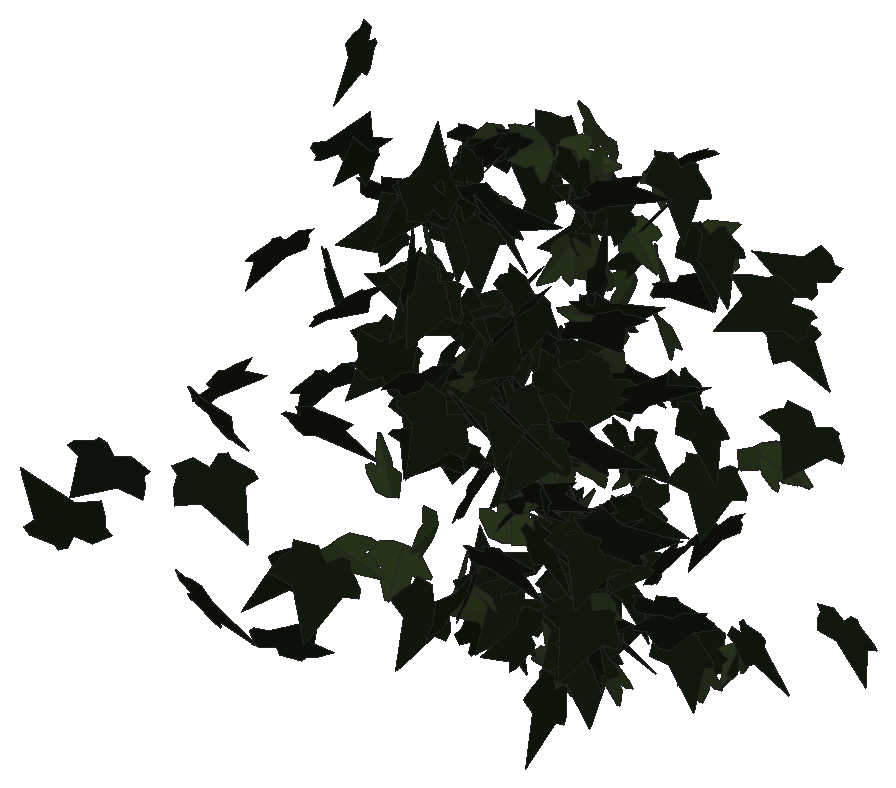
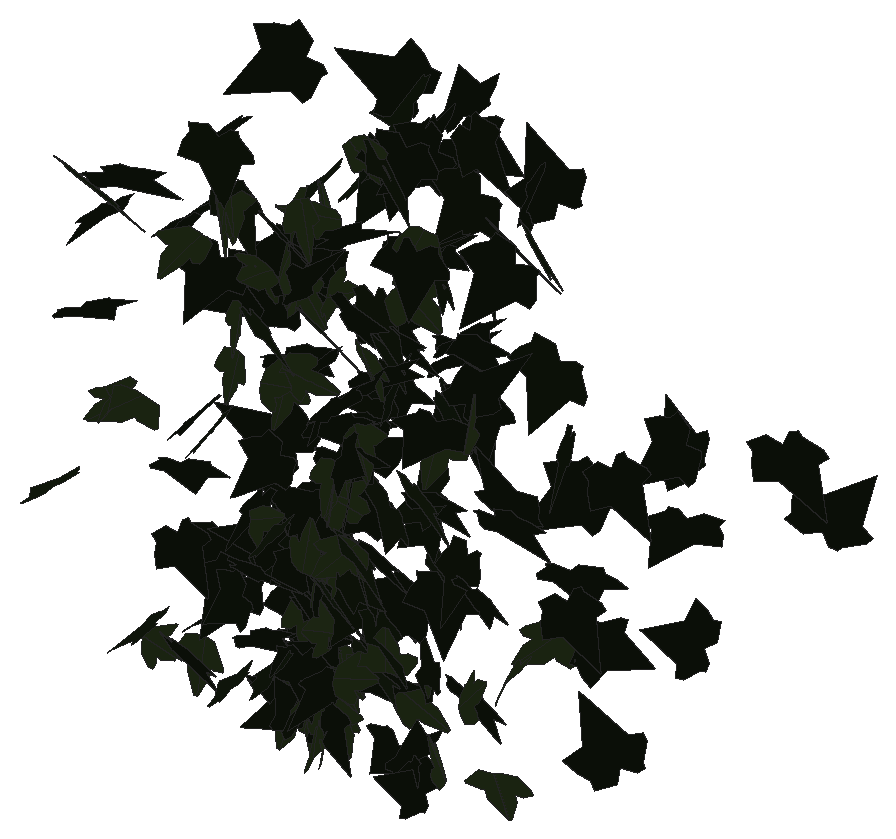
# SketchUp Ruby script. Lengths in millimetres.
U = 1.mm
M = Sketchup.active_model
def pt(a) = Geom::Point3d.new(a.map { |v| v * U })
def face(e, loops, mat)
  f = e.add_face(loops[0].map { |a| pt(a) })
  loops[1..].each { |l| e.add_face(l.map { |a| pt(a) }).erase! }
  f.material = f.back_material = mat if mat
  f
end
# faces: each face lists its corners as indices into pts; further lists are holes
def faces(e, pts, list, mat = nil) = list.each { |f| face(e, (f[0].is_a?(Array) ? f : [f]).map { |l| l.map { |i| pts[i] } }, mat) }
# xy, xz, yz: faces in a plane at the given z, y or x. An outline is a flat list of corners, or four numbers for a rectangle; further outlines are holes
def ring(l) = l.size == 4 ? [[l[0], l[1]], [l[2], l[1]], [l[2], l[3]], [l[0], l[3]]] : l.each_slice(2).to_a
def flat(e, list, mat, &to3) = list.each { |f| face(e, (f[0].is_a?(Array) ? f : [f]).map { |l| ring(l).map { |u, v| to3.(u, v) } }, mat) }
def xy(e, z, list, mat = nil) = flat(e, list, mat) { |x, y| [x, y, z] }
def xz(e, y, list, mat = nil) = flat(e, list, mat) { |x, z| [x, y, z] }
def yz(e, x, list, mat = nil) = flat(e, list, mat) { |y, z| [x, y, z] }
def lines(e, pts, list) = list.each { |a, b| e.add_line(pt(pts[a]), pt(pts[b])) }
# prism: a flat outline (further loops are holes) pulled along v
def prism(e, loops, v, mat = nil)
  f = face(e, loops, mat); d = Geom::Vector3d.new(v.map { |x| x * U })
  f.pushpull(f.normal.samedirection?(d) ? d.length : -d.length)
end
def box(e, o, s, mat = nil) = prism(e, [[o, [o[0] + s[0], o[1], o[2]], [o[0] + s[0], o[1] + s[1], o[2]], [o[0], o[1] + s[1], o[2]]]], [0, 0, s[2]], mat)
def at(x, y, z, deg = 0) = Geom::Transformation.translation(pt([x, y, z])) * Geom::Transformation.rotation(ORIGIN, Z_AXIS, deg.degrees)
def axes(o, x, y, z) = Geom::Transformation.new([*x, 0, *y, 0, *z, 0, *pt(o).to_a, 1])
def part(name) = M.definitions.add(name)
# library, detail: a bought-in or finely detailed component or shape, given as its bounding box
def library(name, o, s) = part(name).tap { |d| box(d.entities, o, s) }
def detail(e, o, s) = box(e.add_group.entities, o, s)
def put(e, d, t, mat = nil) = e.add_instance(d, t).tap { |i| i.material = mat if mat }
def group(e, t, mat = nil) = e.add_group.tap { |g| g.transformation = t; g.material = mat if mat }.entities
root = M.entities
M.materials.add("efeu1").color = [18, 25, 13]
M.materials.add("efeu2").color = [43, 57, 29]
c1 = part("ivyleaf_9")
p = [[39.1,54.8,31.7],[34.5,51.8,30.2],[-5.3,25.2,17.3],[-17.9,28.3,20.9],[-21.6,21.7,17],[-20.2,4.3,5.3],
  [-22.9,-0.3,2.5],[-17.1,-4,-0.6],[-2,-2.1,-1.2],[-0.7,-15.4,-10.1],[16.6,-22.3,-16.7],[21.1,-15.1,-12.5],
  [32.7,-10.7,-11],[46.1,-1.8,-6.6],[30.8,11.2,3.8]]
faces(c1.entities,p,[[0,1,2,3,4,5,6,7,8,9,10,11,12,13,14]],"efeu1")
c2 = part("ivyleaf_10")
p = [[0,12.8,-0.8],[-1.5,51.3,-10.9],[-4.9,51,-11.6],[-13.6,26.5,-7.3],[-13.2,15.9,-4.6],[-21.1,19.3,-7.2],
  [-29.5,16.3,-8.3],[-29.2,8.3,-6.2],[-19.7,-9.8,0.5],[-7.6,-13,4],[1,-12.2,5.8],[-0.4,51.1,-11.1],
  [-1.5,51.1,-10.9],[1,-12.4,5.9],[16.9,-12.4,3.5],[35.1,9.1,-5.1],[35,12.9,-6.1],[20.5,16.4,-4.9],
  [15.8,15,-3.8],[15.3,27.6,-7.1],[12.8,31.3,-7.8]]
faces(c2.entities,p,[[0,1,2,3,4,5,6,7,8,9,10],[11,12,0,13,14,15,16,17,18,19,20]],"efeu2")
put(root,c1,axes([136.9,214.2,2864.8],[0.77182,0.05474,1.30605],[-1.57772,0.23788,0.61645],[-0.23266,-1.43158,0.15237]))
put(root,c1,axes([158.5,636.5,3129.4],[-0.30684,1.08805,-0.78209],[0.11777,-0.77896,-1.11475],[-1.63051,-0.26102,0.06666]))
put(root,c1,axes([184.8,240.9,2983],[0.60978,0.4601,-1.2558],[-1.10179,-0.87272,-0.67919],[-1.20349,1.03209,-0.01449]))
put(root,c1,axes([204.6,673.9,2927.4],[-0.16788,1.09253,-0.72485],[0.08004,-0.72218,-1.10096],[-1.59756,-0.15099,0.02101]))
put(root,c1,axes([229.9,398.1,3039.6],[0.65237,0.88713,0.88336],[0.57443,0.74753,-1.03574],[-1.41521,0.71236,-0.01321]))
put(root,c1,axes([253.2,613,3131.7],[0.91465,-0.33065,-1.03128],[-1.14312,0.43093,-0.81933],[0.66254,1.19997,0.01007]))
put(root,c1,axes([235.6,386.8,2918.7],[-0.41955,-0.88281,-1.0429],[0.48535,0.96414,-0.94732],[1.59476,-0.52568,0.01394]))
put(root,c1,axes([216.5,376.4,2726.7],[1.0554,-0.66857,0.9113],[0.86392,-0.57383,-1.09321],[1.07471,1.11784,-0.01614]))
put(root,c1,axes([234.5,386.1,3004.3],[1.49533,-0.3407,-0.54294],[0.66687,-0.05634,1.26933],[-0.40842,-1.33937,0.08471]))
put(root,c1,axes([272.6,670.1,3457.6],[-1.25435,0.37299,-0.69527],[0.78343,-0.26797,-1.09337],[-0.55928,-1.2119,0.02778]))
put(root,c1,axes([247.5,515.9,2598.5],[1.5333,0.5588,0.01046],[-0.02051,0.01206,1.37531],[0.68155,-1.25679,0.01784]))
put(root,c2,axes([293.4,689.6,2785.9],[-0.01942,1.10423,-0.61306],[-0.34661,0.59426,1.07776],[1.50137,0.15148,0.24088]))
put(root,c2,axes([281.3,728.5,2655.5],[1.47576,0.32086,-0.1164],[-0.12947,-0.05384,-1.25123],[-0.39578,1.21403,-0.02472]))
put(root,c1,axes([302.5,495.3,2756],[-0.27263,0.16305,-1.32385],[0.36508,-1.30195,-0.21087],[-1.58582,-0.32776,0.17905]))
put(root,c1,axes([327.3,671.1,3014.8],[-1.58771,-0.34703,-0.02695],[0.02402,0.03073,-1.34665],[0.42397,-1.30131,-0.02462]))
put(root,c1,axes([334.5,714.7,2919.2],[-1.1837,-0.20215,-0.69409],[0.85266,0.03471,-0.98709],[0.22549,-1.19245,0.08893]))
put(root,c1,axes([313,491.2,2980.5],[1.70691,0.20299,0.32695],[0.39528,0.04395,-1.41375],[-0.25336,1.43613,-0.00294]))
put(root,c2,axes([334.8,725.4,3152],[-0.91571,0.77432,0.53057],[0.45827,-0.3748,1.07837],[1.04947,0.83929,-0.00793]))
put(root,c2,axes([339.4,535.7,2769.8],[-0.88971,-0.46879,-0.88039],[0.97357,0.38003,-0.86339],[0.72999,-1.07819,0.07847]))
put(root,c1,axes([341.5,622.6,2998.7],[-0.93859,0.40157,1.0261],[1.02223,-0.59954,0.86286],[0.87303,1.13372,0.09285]))
put(root,c1,axes([361,501.6,3162.6],[0.62636,1.33083,0.45001],[0.08995,0.45293,-1.4236],[-1.71156,0.51083,0.08987]))
put(root,c2,axes([358.1,699.1,2734.2],[0.01988,0.01032,1.20059],[0.61594,-1.08944,0.00251],[1.32898,0.50477,-0.01913]))
put(root,c1,axes([378.1,676.8,2938.7],[1.29505,-0.02891,-0.80604],[-0.97157,0.17363,-1.05499],[0.15598,1.3215,0.12098]))
put(root,c2,axes([379.8,729,2635.2],[0.73316,-0.99484,0.15197],[-0.08902,0.13346,1.16224],[-1.22455,-0.60533,0.00649]))
put(root,c1,axes([371.2,491.6,3406],[1.21168,0.88272,0.41487],[-0.38302,-0.27126,1.32874],[1.1266,-1.0416,0.00555]))
put(root,c1,axes([389.4,434.8,2807],[-1.25164,-0.91954,-0.43292],[0.44036,0.24538,-1.3766],[1.15912,-1.08616,0.05551]))
put(root,c1,axes([404.5,685.8,2886.7],[1.06678,0.59143,-0.70397],[-0.72278,-0.38051,-1.05555],[-0.85781,1.05612,0.01392]))
put(root,c1,axes([414.2,625.9,3142.8],[0.02648,-0.01708,1.38171],[-1.38884,-0.78349,0.0082],[0.95555,-1.1383,-0.02637]))
put(root,c1,axes([392.8,522.4,3415.1],[0.02963,-0.43729,-1.21261],[0.99483,-0.93412,0.35319],[-1.218,-0.7736,0.25898]))
put(root,c1,axes([389.7,562.1,3329.3],[1.67986,0.4873,-0.08396],[-0.09219,-0.03812,-1.46058],[-0.59617,1.37896,-0.0107]))
put(root,c1,axes([427.4,735,2640.3],[-0.67316,-0.80181,0.80469],[0.55796,0.66209,0.97332],[-1.2686,0.71667,0.00109]))
put(root,c1,axes([431.9,608.8,2686.9],[-1.55648,-0.05865,-0.52322],[0.63718,0.03237,-1.27713],[0.08118,-1.37855,-0.00773]))
put(root,c1,axes([420.4,714.1,2582.9],[0.04994,-0.01153,1.22765],[1.0354,0.88784,-0.01996],[-1.08229,0.84884,0.03755]))
put(root,c1,axes([455.2,688.5,3021.2],[-0.74037,0.92777,0.43428],[-0.33707,0.33782,-1.10778],[-1.20343,-0.6654,0.0431]))
put(root,c1,axes([468.4,494.2,3323.5],[-1.42603,0.67788,0.32122],[-0.36271,0.12739,-1.35069],[-0.84022,-1.2055,0.03789]))
put(root,c1,axes([469.1,623.6,3329.9],[-0.62842,0.24837,-1.19726],[-1.28895,0.5636,0.57147],[0.75097,1.17521,-0.02103]))
put(root,c1,axes([434.9,667.7,3118.9],[-0.55013,-0.7202,-1.03942],[0.62884,0.90301,-0.84929],[1.40877,-0.68433,-0.02679]))
put(root,c1,axes([454.1,686.7,3379.4],[0.95125,0.81246,-0.47219],[-0.43252,-0.3139,-1.12552],[-1.06173,0.85579,0.03545]))
put(root,c1,axes([462.1,585.1,3197.8],[-1.52178,-0.55158,-0.06751],[0.06011,0.05545,-1.36353],[0.67527,-1.24796,-0.03075]))
put(root,c1,axes([463.4,659.5,2991.2],[-1.3795,-0.3644,-0.00526],[0.00562,0.00284,-1.188],[0.44458,-1.13074,-0.00129]))
put(root,c2,axes([489,658.2,2676],[-0.54557,-0.10103,1.05054],[-1.22859,-0.30051,-0.45757],[0.38522,-1.1015,0.02848]))
put(root,c1,axes([473.9,535.5,3082.6],[0.4258,1.23479,-0.40666],[-0.20004,-0.37589,-1.28207],[-1.57337,0.38196,0.05295]))
put(root,c2,axes([468.9,623,3061.5],[-0.64221,-1.05806,-0.43899],[0.24261,0.39139,-1.18177],[1.37631,-0.5627,0.00347]))
put(root,c2,axes([485.6,666,3295.5],[-0.75887,-0.77137,0.76488],[-0.53741,-0.62658,-0.99012],[1.21144,-0.76116,0.03992]))
put(root,c1,axes([467.7,577.8,3198.2],[-0.62407,-1.18911,0.42605],[-0.13223,-0.41664,-1.29299],[1.53533,-0.51923,0.06182]))
put(root,c1,axes([486.5,493.1,3235.3],[0.00813,0.26994,1.37358],[-0.10834,1.37091,-0.26898],[-1.70438,-0.08586,0.02365]))
put(root,c2,axes([469.6,661.1,3382.7],[-0.51677,-0.91674,-0.75887],[0.43496,0.67076,-1.00931],[1.38522,-0.55262,0.03382]))
put(root,c1,axes([457.4,724.2,2645.4],[-0.63324,-0.1734,-1.15273],[1.32539,0.38553,-0.54717],[0.51561,-1.20397,-0.00919]))
put(root,c2,axes([475.6,724.7,2762.7],[1.31573,0.66947,-0.05661],[0.04977,0.04161,1.26929],[0.81815,-1.07915,0.01383]))
put(root,c1,axes([471.7,630.6,2690.7],[0.08567,0.81467,0.81948],[-0.20399,-0.80519,0.81479],[1.3949,-0.16778,0.06883]))
put(root,c1,axes([493.2,574.6,3095.2],[-1.24934,0.8159,-0.63929],[0.59082,-0.41793,-1.30915],[-1.11805,-1.13256,0.02255]))
put(root,c1,axes([498.1,712.4,2814],[-0.65809,1.07353,-0.03794],[0.012,-0.03752,-1.20141],[-1.31047,-0.53945,0.00805]))
put(root,c1,axes([458.6,636.7,2990.8],[1.43342,-0.70007,-0.01095],[0.02718,0.05877,-1.36629],[0.85375,1.17352,0.06189]))
put(root,c1,axes([497.2,688.8,2978.1],[-0.01566,0.91777,0.91135],[-0.16083,0.90572,-0.91396],[-1.56972,-0.10195,0.08455]))
put(root,c2,axes([495.1,788.7,2762.1],[0.02768,-0.34689,1.0574],[-0.00072,-1.05763,-0.34695],[1.35768,0.00651,-0.02174]))
put(root,c1,axes([492.4,507.5,3376.6],[0.73502,1.12768,0.73941],[0.34552,0.68597,-1.27695],[-1.60845,0.66268,0.06358]))
put(root,c1,axes([515.7,745.4,2938],[-0.62625,0.96456,0.35543],[-0.2695,0.28449,-1.09109],[-1.22482,-0.55578,0.05835]))
put(root,c1,axes([536.5,734.7,3282.8],[-1.07698,0.04613,-0.82764],[-1.00803,-0.14579,0.87318],[-0.08098,1.20126,0.13776]))
put(root,c1,axes([500.4,589.9,3326.1],[-0.24615,-1.39197,0.02568],[-0.05008,-0.01999,-1.40601],[1.69775,-0.20241,-0.03775]))
put(root,c1,axes([532.8,682.3,2733.8],[-0.35314,1.00279,0.71441],[-0.53194,0.60284,-1.02285],[-1.40478,-0.48037,0.20773]))
put(root,c1,axes([526.2,476.6,3445.9],[-0.74835,1.00067,-0.76076],[0.43701,-0.67226,-1.17308],[-1.46997,-0.70929,0.03855]))
put(root,c1,axes([522,751.4,2896.5],[-0.86446,0.42285,-0.78669],[0.58855,-0.66391,-0.79137],[-0.917,-0.82473,0.23371]))
put(root,c1,axes([526.7,568.7,2904.9],[-0.4203,0.64939,-1.09967],[-0.87484,0.84413,0.72314],[1.28927,0.78448,0.13219]))
put(root,c1,axes([533.4,478.9,3027.2],[0.70862,0.57847,-0.99218],[-0.89324,-0.67013,-0.81932],[-1.07954,0.9342,0.02664]))
put(root,c1,axes([530.6,706.3,2869.5],[0.13504,0.069,1.1975],[-0.0964,1.20039,-0.06186],[-1.46019,-0.07287,0.11483]))
put(root,c1,axes([531.8,677,2697.5],[-1.33744,-0.5986,0.03158],[-0.03425,-0.01448,-1.24904],[0.7305,-1.09662,-0.00075]))
put(root,c1,axes([536.2,696.6,2908.9],[-1.47572,0.01465,-0.26376],[0.32108,-0.03981,-1.20917],[-0.0278,-1.23739,0.03578]))
put(root,c2,axes([513.8,758.2,2937.6],[-1.00947,-0.31894,-0.70837],[0.82737,0.20825,-0.88593],[0.4623,-1.06914,0.03875]))
put(root,c1,axes([528.2,581.4,3320],[-0.98778,-0.79475,-0.74508],[0.65156,0.51954,-1.13453],[1.15838,-0.96993,0.0028]))
put(root,c1,axes([531.3,745.7,3069],[-0.20372,0.2072,-1.16645],[1.0102,-0.82206,-0.26456],[-1.03369,-0.84422,-0.02867]))
put(root,c1,axes([543.1,657.8,3144.8],[-0.75179,-0.87674,0.64164],[-0.35899,-0.57541,-1.06884],[1.27593,-0.67848,0.07734]))
put(root,c1,axes([549.5,466.8,3424.1],[-0.08227,0.31516,-1.46174],[0.33399,-1.43589,-0.32222],[-1.79347,-0.28185,0.00705]))
put(root,c1,axes([525.2,613.4,2792.1],[1.6516,0.2622,-0.04909],[-0.06058,-0.00181,-1.3789],[-0.31975,1.35466,0.00766]))
put(root,c2,axes([560.2,736.6,2665.1],[-1.22932,-0.19474,0.58965],[-0.69685,-0.15027,-1.02572],[0.29722,-1.15777,0.03396]))
put(root,c1,axes([563.8,483.8,2774],[-0.38003,1.11855,0.63387],[-0.21874,0.60804,-1.16108],[-1.55319,-0.35932,0.00843]))
put(root,c1,axes([564.2,729.3,3382],[-0.89361,-0.31815,0.86652],[-0.79635,-0.60363,-0.77339],[0.79628,-0.96072,0.19897]))
put(root,c1,axes([538.7,703,2831.9],[1.50721,0.24901,-0.29936],[-0.40838,0.17039,-1.23968],[-0.24269,1.2597,0.22686]))
put(root,c1,axes([567.5,740.4,2660.6],[0.39621,0.26357,-1.06223],[-1.26055,-0.29149,-0.38822],[-0.44024,1.07183,0.15563]))
put(root,c1,axes([545.7,531.8,3434.3],[0.73306,0.91157,0.89309],[0.63156,0.72816,-1.09151],[-1.42305,0.79274,-0.02436]))
put(root,c2,axes([558.1,747.3,2792.4],[0.35423,-0.56349,0.97249],[-0.32301,0.94186,0.62479],[-1.33263,-0.37808,0.10706]))
put(root,c1,axes([561.2,576.9,3451.6],[0.83956,1.04968,-0.22079],[-0.15834,-0.17891,-1.25511],[-1.29902,0.70022,0.01029]))
put(root,c1,axes([552,740.5,2719.3],[0.12016,-0.50179,-1.10592],[-0.20053,1.09383,-0.51094],[1.46798,0.19049,0.02073]))
put(root,c2,axes([567,758.6,2611.2],[-0.1433,1.05571,-0.48115],[-0.05793,0.47883,1.06221],[1.41424,0.12658,-0.00524]))
put(root,c2,axes([564.3,653.3,3170.2],[1.27326,-0.66297,-0.14136],[-0.15068,0.06921,-1.2364],[0.81317,1.05091,-0.00776]))
put(root,c1,axes([580.2,592.8,3444.9],[-0.48915,1.2023,0.0323],[-0.01564,0.02977,-1.26739],[-1.46725,-0.40114,0.00274]))
put(root,c1,axes([587.9,713,2833.7],[-1.13152,0.73043,0.11664],[-0.11019,0.07384,-1.18057],[-0.89567,-0.93186,-0.00212]))
put(root,c2,axes([579.8,700.1,2860.5],[0.38363,-0.24174,1.10037],[-0.7954,0.89265,0.38242],[-1.12093,-0.71615,0.10523]))
put(root,c1,axes([579.3,591.5,3066],[0.17064,-1.03299,0.86864],[0.03121,0.87517,1.03663],[-1.6463,-0.09048,0.10968]))
put(root,c1,axes([587,587.2,3167.9],[-1.50474,-0.16173,0.02804],[-0.03304,-0.00914,-1.24394],[0.19751,-1.23368,0.00554]))
put(root,c1,axes([571.5,463.7,3085.9],[-0.66515,-1.24172,0.59558],[-0.28001,-0.54967,-1.3561],[1.65664,-0.59146,0.00992]))
put(root,c1,axes([591.4,601.4,3223],[-0.62597,1.23624,-0.04847],[-0.00009,-0.05251,-1.33834],[-1.50937,-0.51269,0.02018]))
put(root,c1,axes([598.6,733.5,3250.5],[-1.10133,0.64888,0.27047],[-0.3209,0.09646,-1.10934],[-0.79535,-0.93743,0.07306]))
put(root,c2,axes([576.2,729,2661.3],[-1.41867,-0.47732,-0.17273],[0.24489,-0.03584,-1.25231],[0.56881,-1.17505,0.10836]))
put(root,c2,axes([567.3,746.3,2616.4],[0.00396,0.02338,-1.17165],[0.35424,-1.13513,-0.02185],[-1.38511,-0.29024,-0.00894]))
put(root,c1,axes([581.3,514.3,3416.6],[-0.19568,-0.16384,1.30254],[-0.64548,-1.19287,-0.21519],[1.46579,-0.54717,0.07912]))
put(root,c1,axes([585.2,420.6,3431.9],[-0.66901,-0.83607,1.09748],[0.86473,0.84251,0.99599],[-1.44409,0.89183,0.08796]))
put(root,c2,axes([586.4,644.6,3035.4],[-0.16503,-1.21402,0.08141],[-0.00582,-0.08138,-1.22152],[1.48442,-0.13529,0.00426]))
put(root,c1,axes([613.7,703.2,2779.5],[-0.26167,0.37712,1.0581],[-1.16877,0.50106,-0.37278],[-0.71558,-0.95631,0.22194]))
put(root,c2,axes([606.4,742.5,3415],[-1.14686,0.31079,0.73922],[-0.85526,0.23453,-0.99009],[-0.475,-1.17266,-0.0021]))
put(root,c2,axes([596.9,742.4,2886],[-1.36344,0.22641,0.0382],[0.04057,-0.0282,1.14008],[0.27717,1.11787,0.02102]))
put(root,c2,axes([613,608.3,3447.7],[0.95307,-0.22671,-0.94822],[-1.07693,0.35136,-0.81126],[0.50495,1.17727,0.05952]))
put(root,c1,axes([615.2,715.3,2822.8],[0.13167,0.09878,-1.11888],[-1.3702,-0.00721,-0.10897],[-0.02036,1.12405,0.09763]))
put(root,c1,axes([603.5,581.7,3167.7],[-1.08714,-0.81659,0.25515],[-0.23065,-0.17134,-1.20867],[1.01794,-0.91093,-0.00138]))
put(root,c2,axes([616.4,721.1,2671.4],[1.05435,-0.01464,-0.74475],[-0.90394,0.10058,-0.86177],[0.09359,1.13641,0.06668]))
put(root,c1,axes([600.6,573,3082.6],[-1.2669,-0.75888,-0.53591],[0.52725,0.3169,-1.28618],[1.00331,-1.12478,-0.0008]))
put(root,c1,axes([617.1,753.2,3294.7],[-0.25645,0.0878,1.18135],[-1.08886,-0.80066,-0.0993],[0.9503,-0.89371,0.20502]))
put(root,c2,axes([603,689,2630.8],[-0.7108,0.99678,-0.04156],[0.02573,-0.03581,-1.15456],[-1.21685,-0.583,-0.00014]))
put(root,c1,axes([590.9,583,3003.1],[0.33459,-0.11233,-1.34913],[-0.1075,1.37213,-0.13216],[1.64813,0.1123,0.26527]))
put(root,c1,axes([614.7,727.4,2725],[0.16149,1.08542,-0.29619],[-0.04199,-0.29419,-1.09346],[-1.37198,0.13676,-0.0014]))
put(root,c1,axes([615.2,647.7,3001.2],[-1.35327,-0.64378,-0.16904],[0.15326,0.12013,-1.28188],[0.79744,-1.1156,-0.04049]))
put(root,c1,axes([630.1,552.2,3154.2],[-0.66576,1.1926,0.22534],[-0.16601,0.18539,-1.31072],[-1.47138,-0.56054,0.04592]))
put(root,c2,axes([609.7,672.5,3256.5],[0.13266,0.42943,-1.1541],[-0.28029,-1.13117,-0.44255],[-1.47593,0.25342,-0.01969]))
put(root,c2,axes([613.5,665.5,2980.4],[-1.32998,0.52447,0.12319],[-0.135,0.05415,-1.20975],[-0.64325,-1.09575,-0.00082]))
put(root,c2,axes([616.8,649,2928.1],[-0.3462,-0.71139,0.96788],[-0.09838,-0.98099,-0.74467],[1.46214,-0.23444,0.17906]))
put(root,c1,axes([618.2,615.7,2945.4],[0.55631,-0.29484,-1.13077],[-1.19625,0.56379,-0.54241],[0.77557,1.08107,-0.02553]))
put(root,c2,axes([607.4,706.7,2845.4],[-0.34705,0.68872,-0.88462],[0.08629,-0.89981,-0.72329],[-1.36503,-0.23199,0.17918]))
put(root,c2,axes([598,789.1,3341.9],[0.00503,0.02264,1.17313],[0.89678,-0.91445,0.01506],[1.11577,0.73487,-0.0174]))
put(root,c2,axes([622.5,615.5,2963.2],[-0.1766,0.24372,1.22244],[-0.69003,1.08383,-0.28306],[-1.35517,-0.58363,-0.01518]))
put(root,c2,axes([639.5,715.1,3147.6],[0.27846,0.05034,-1.15018],[-1.39188,0.16707,-0.21909],[0.18828,1.16064,0.08142]))
put(root,c2,axes([641.8,620.8,2666.8],[-0.59082,0.05314,1.09712],[-1.32193,0.17343,-0.48669],[-0.21966,-1.18664,-0.022]))
put(root,c1,axes([602.9,661.6,3093.8],[0.40279,-1.10305,-0.62909],[-0.1927,0.60928,-1.15121],[1.53716,0.36541,0.02053]))
put(root,c1,axes([603.1,598.3,2915.6],[1.20407,0.78539,0.59876],[0.56476,0.37986,-1.26128],[-1.06432,1.09009,0.00811]))
put(root,c1,axes([617.1,744.8,2643.9],[-0.22091,-0.57667,0.95215],[0.81366,0.71615,0.56058],[-1.08733,0.65307,0.22604]))
put(root,c1,axes([621.2,663.7,3051.9],[-0.8082,-0.97908,-0.01181],[0.00984,0.0088,-1.18213],[1.19452,-0.66251,0.00175]))
put(root,c2,axes([611,737.9,2688.4],[1.31359,-0.10545,0.3278],[0.4035,0.01727,-1.08083],[0.1169,1.12537,0.0473]))
put(root,c2,axes([634.1,640.1,2951.2],[-0.7811,0.67585,0.72772],[-0.63431,0.50961,-0.93072],[-1.03234,-0.8245,0.02126]))
put(root,c1,axes([626.1,699.2,2732.5],[-0.92584,-0.90505,0.01312],[-0.00483,-0.01379,-1.1811],[1.10426,-0.75888,0.00583]))
put(root,c1,axes([625.5,549.2,3173.5],[-0.46734,-0.79546,1.00401],[-0.44902,-0.9354,-0.88152],[1.49683,-0.52896,0.04903]))
put(root,c1,axes([635.6,708.5,2857.7],[-0.06189,1.09817,-0.3424],[0.05915,-0.34039,-1.0989],[-1.40214,-0.06284,-0.03124]))
put(root,c2,axes([598.6,695.5,3387.7],[0.13614,-0.35015,-1.1133],[1.41844,0.13053,0.07548],[0.12372,-1.11124,0.35967]))
put(root,c1,axes([598.8,560.3,3054.1],[1.16504,-0.66061,0.53058],[0.53632,-0.29713,-1.16117],[0.88369,1.05126,0.00523]))
put(root,c2,axes([649.5,622,2652.5],[-1.16809,-0.05087,0.76789],[-0.91848,-0.1922,-0.95143],[0.19464,-1.21219,0.11863]))
put(root,c2,axes([635.9,660.1,3396.8],[0.56365,-0.90969,-0.6142],[-0.24803,0.58394,-1.0178],[1.31593,0.49971,0.07124]))
put(root,c2,axes([626.3,785,3163.6],[0.07642,-0.53668,1.05015],[0.41132,-0.99959,-0.53095],[1.37874,0.32795,0.10019]))
put(root,c1,axes([643.2,592.2,3017.3],[-1.30032,-0.73271,0.05135],[-0.03282,-0.0515,-1.29311],[0.8955,-1.06583,0.02718]))
put(root,c1,axes([659.1,533.5,2748.9],[-1.19431,0.88801,0.16646],[-0.15803,0.10496,-1.32166],[-1.09085,-0.98743,0.00922]))
put(root,c1,axes([626.2,786.8,2923.6],[-0.09394,-0.86358,0.65064],[0.1325,-0.65516,-0.85673],[1.31245,0.00433,0.13306]))
put(root,c1,axes([614.8,744.5,2658.4],[1.27298,-0.39876,0.2221],[0.26102,-0.06223,-1.11688],[0.49189,1.06498,0.0179]))
put(root,c2,axes([661.9,675.6,3253.5],[-0.9258,-0.02382,0.91956],[-1.12217,0.0069,-0.75889],[0.012,-1.19222,-0.02277]))
put(root,c1,axes([615.9,710.4,2636.9],[0.02243,-0.04802,1.19794],[1.45297,0.13843,-0.01273],[-0.1681,1.19006,0.04982]))
put(root,c1,axes([629.6,762.3,3042.8],[1.31079,0.25417,0.03851],[0.04765,0.00217,-1.10405],[-0.30998,1.07511,-0.00687]))
put(root,c1,axes([628.9,587.5,2871.2],[0.95095,-0.96786,-0.28075],[-0.20834,0.22294,-1.24269],[1.21168,0.79793,0.00667]))
put(root,c1,axes([626.7,774.8,2716.6],[0.56405,-1.06208,0.29567],[0.18959,-0.25463,-1.15767],[1.33159,0.48614,0.03959]))
put(root,c2,axes([651.5,684.6,3395.5],[-0.47947,1.02545,0.52096],[-0.37542,0.43672,-1.09178],[-1.35208,-0.4849,0.11841]))
put(root,c1,axes([668.1,764.8,3240.5],[-0.96938,0.80281,0.0977],[-0.10754,0.05017,-1.12921],[-0.98077,-0.79899,0.02725]))
put(root,c1,axes([655.5,781.8,2768.1],[-0.96985,-0.67298,0.20649],[-0.15347,-0.17066,-1.04045],[0.84499,-0.80341,0.04804]))
put(root,c2,axes([656.2,693.2,3241.5],[-0.58766,1.05831,-0.15975],[-0.1088,0.13489,1.1625],[1.30122,0.48924,0.02506]))
put(root,c2,axes([652.3,706.2,2627.6],[-1.40121,0.37342,-0.02742],[0.03743,0.0057,-1.20762],[-0.45526,-1.14884,-0.0149]))
put(root,c1,axes([655.1,653.2,2713.5],[-0.98755,-0.86204,0.34152],[-0.09772,-0.38664,-1.1658],[1.12699,-0.78891,0.19818]))
put(root,c1,axes([640.7,661.4,3406.3],[0.29206,-1.14543,0.32709],[0.15969,-0.30632,-1.16848],[1.44449,0.26546,0.06304]))
put(root,c2,axes([663,651.7,2750.7],[-0.91433,-1.01351,-0.09522],[0.06894,0.07664,-1.26051],[1.24001,-0.75158,-0.00013]))
put(root,c1,axes([645.5,656.9,3134.7],[0.40082,-0.9976,-0.52329],[-0.13038,0.51503,-1.04895],[1.36815,0.34135,0.05334]))
put(root,c1,axes([693.2,646.9,2677.1],[-1.20128,0.63925,0.6458],[-0.88612,0.01851,-1.12576],[-0.66615,-1.17739,0.33293]))
put(root,c2,axes([661.5,701.2,3115],[-0.27568,-0.99732,-0.62733],[0.20329,0.60529,-1.02231],[1.42298,-0.27969,0.02451]))
put(root,c1,axes([688.9,765,2854.5],[-1.10453,0.28035,0.55794],[-0.71886,-0.05838,-0.9268],[-0.2521,-1.06186,0.19826]))
put(root,c1,axes([667.1,610.1,2856.6],[1.27356,0.72586,-0.30831],[-0.3223,-0.16006,-1.27132],[-0.90653,1.07665,0.01886]))
put(root,c1,axes([644.3,459.7,3442.6],[1.00273,-1.09433,0.36045],[0.23571,-0.30559,-1.36832],[1.38573,0.84384,-0.02807]))
put(root,c2,axes([675.9,750.7,2927.2],[-0.26983,0.40927,-1.00794],[-0.36521,-1.01174,-0.34513],[-1.27595,0.20304,0.31194]))
put(root,c1,axes([700.6,690.7,3342.8],[-1.28898,0.57307,0.20236],[-0.21486,0.09972,-1.20195],[-0.70963,-1.07112,-0.00364]))
put(root,c1,axes([675.3,741.8,2953.7],[0.45259,-0.47658,-0.94765],[-0.57398,0.82586,-0.5995],[1.15985,0.59467,0.07311]))
put(root,c1,axes([689.8,640.8,3240.4],[-0.00997,-0.61423,1.11132],[0.49538,1.05172,0.58427],[-1.46777,0.35914,0.18965]))
put(root,c1,axes([697.5,612.1,2739.4],[0.55347,1.17888,-0.0892],[-0.05272,-0.07895,-1.2631],[-1.44138,0.45556,0.01195]))
put(root,c2,axes([699,761.5,3235.1],[-0.97313,0.80045,0.26737],[-0.32338,0.11165,-1.12504],[-0.97748,-0.83382,0.10602]))
put(root,c1,axes([676.9,706.4,2843],[1.18237,-0.49051,-0.43138],[0.48392,-0.17132,1.08594],[-0.63317,-1.0469,0.02441]))
put(root,c1,axes([681.5,624.9,2683.2],[-0.80927,-0.76295,-0.71327],[0.96441,0.18549,-0.93357],[0.83278,-0.95622,0.388]))
put(root,c1,axes([671.5,606.9,2860.2],[0.73483,1.10718,-0.39853],[0.24957,0.34236,1.26031],[1.41373,-0.63593,-0.01534]))
put(root,c2,axes([680.7,728.6,3290.8],[-0.99877,-0.01053,-0.84488],[0.91453,-0.55189,-0.71948],[-0.47567,-1.03897,0.39074]))
put(root,c1,axes([661.6,437,3444.6],[0.67639,-0.43722,1.30787],[1.49219,-0.49516,-0.68402],[0.77706,1.33143,0.1751]))
put(root,c1,axes([709.4,600.1,2727.8],[0.87733,-0.28563,-1.09556],[-1.15118,0.56605,-0.76695],[0.76333,1.18194,0.10255]))
put(root,c1,axes([713.2,635.6,3112.7],[-1.17509,-0.94532,0.21405],[-0.10725,-0.21532,-1.34651],[1.17762,-0.9629,0.09096]))
put(root,c1,axes([678.3,705.7,2868.6],[0.62137,0.08396,-1.03386],[0.9537,0.72598,0.44406],[0.83178,-0.89511,0.26318]))
put(root,c1,axes([693.8,782.4,2675.9],[0.19399,-0.96979,0.43911],[0.23034,-0.41125,-0.97664],[1.27818,0.2213,0.10935]))
put(root,c2,axes([714.2,749.2,3151.7],[-1.19929,0.58571,0.15816],[-0.16551,0.0813,-1.14429],[-0.72142,-0.99234,-0.0004]))
put(root,c1,axes([719.8,420,3300.2],[0.30502,1.19564,0.84834],[0.22523,0.82806,-1.22147],[-1.77432,0.31065,-0.00921]))
put(root,c2,axes([710.7,754.1,3389.9],[0.01275,-1.16504,0.22926],[0.4415,-0.21523,-1.11027],[1.37968,0.07964,0.35317]))
put(root,c1,axes([686.9,649.8,3197.6],[0.27759,-0.37692,1.15478],[1.4588,-0.1375,-0.28049],[0.26111,1.16893,0.33937]))
put(root,c1,axes([716.3,732.9,2785.3],[0.27198,0.64113,0.94208],[0.45805,0.86501,-0.67753],[-1.31261,0.4347,-0.04123]))
put(root,c1,axes([721.4,507,2697.4],[-1.37287,0.13238,-0.89166],[1.06008,-0.22032,-1.12931],[-0.29272,-1.41874,0.09218]))
put(root,c1,axes([720.3,606.2,2890.3],[-1.00426,-1.11408,-0.13571],[0.11145,0.10123,-1.38513],[1.36468,-0.82811,0.01326]))
put(root,c1,axes([726.3,582.2,2787.1],[-1.4266,-0.58558,-0.35614],[0.43689,0.0785,-1.30488],[0.71295,-1.21985,0.08699]))
put(root,c1,axes([710.3,475.8,3310.5],[-0.14094,-1.26306,0.82528],[0.15608,-0.83291,-1.25683],[1.83407,-0.02618,0.17038]))
put(root,c2,axes([727,761.4,3380.8],[0.97953,-0.84405,-0.21376],[-0.00316,0.28846,-1.14871],[1.06224,0.77919,0.1937]))
put(root,c1,axes([733,576,3235.6],[0.99967,1.17922,-0.02418],[-0.01526,-0.02075,-1.43596],[-1.43887,0.8195,-0.00157]))
put(root,c1,axes([727.1,772.4,3058.3],[0.67585,-0.95704,-0.25403],[-0.14368,0.22533,-1.10576],[1.19945,0.56626,0.01068]))
put(root,c1,axes([760.8,692.7,3368.6],[-0.45183,1.26206,-0.0771],[0.02269,-0.07489,-1.31528],[-1.54242,-0.37081,0.00323]))
put(root,c1,axes([779.1,700.6,3445.5],[0.31916,1.25673,-0.14425],[-0.27524,-0.09859,-1.26807],[-1.51853,0.282,0.19952]))
put(root,c1,axes([761,678.8,2772.4],[1.40672,0.53657,-0.16756],[-0.18108,-0.07818,-1.27176],[-0.66146,1.16254,-0.00818]))
put(root,c1,axes([797.4,763,2864],[-0.24695,0.99267,-0.67148],[0.16461,-0.65779,-1.0131],[-1.45281,-0.24327,-0.00065]))
put(root,c1,axes([782.8,696.4,3259.7],[1.05643,0.95595,0.02826],[0.02044,0.02296,-1.28983],[-1.16658,0.86608,0.003]))
put(root,c2,axes([794.4,719.9,2673.9],[-1.47901,0.31374,0.17194],[-0.21314,0.01097,-1.25181],[-0.38089,-1.22439,0.03284]))
put(root,c1,axes([808.8,755.4,2688.8],[-1.82384,0.20993,-0.28935],[0.54942,-0.03383,-0.98064],[-0.40127,-1.00046,-0.02756]))
put(root,c2,axes([786.7,747.6,3308.5],[0.5816,0.80066,0.82643],[0.32139,0.79484,-0.92203],[-1.36653,0.5277,0.13488]))
put(root,c1,axes([763.3,565.3,2920.1],[0.44302,-0.28023,1.35676],[1.60803,-0.36211,-0.42756],[0.52056,1.35704,0.16608]))
put(root,c1,axes([788.3,737.6,3039.7],[0.28223,-1.21427,0.00058],[-0.00057,-0.00068,-1.23611],[1.48141,0.23133,-0.00058]))
put(root,c1,axes([795,685.9,3440.3],[-0.02535,-1.32132,0.08677],[0.0108,-0.08692,-1.32145],[1.61545,-0.02015,0.0102]))
put(root,c1,axes([793.5,691.4,2717.6],[0.05833,-1.27209,0.07864],[0.19878,-0.07195,-1.26292],[1.54215,0.05739,0.15981]))
put(root,c1,axes([791.7,507.2,3481.8],[1.22969,0.72247,0.8533],[0.76839,0.58234,-1.23702],[-1.12704,1.1853,0.08765]))
put(root,c1,axes([808.1,741.9,2959.4],[-0.9964,-0.85302,-0.37641],[0.44839,0.16533,-1.17215],[1.04539,-0.88396,0.144]))
put(root,c1,axes([826.9,629.7,2791.3],[0.56315,1.13972,-0.5279],[-0.36116,-0.44786,-1.22577],[-1.4892,0.53961,0.09764]))
put(root,c1,axes([811.9,716.2,3325.7],[0.14384,-1.23943,-0.01792],[-0.02732,0.01587,-1.24485],[1.51202,0.1182,-0.02079]))
put(root,c1,axes([807.1,567.8,3149.3],[0.99622,0.46889,1.0733],[0.96415,0.7451,-0.92677],[-1.05464,1.1241,0.1666]))
put(root,c1,axes([813.9,727.8,3327.6],[0.07858,-1.26542,-0.13106],[0.15745,0.13705,-1.25983],[1.54406,0.05042,0.13513]))
put(root,c1,axes([799.1,455.4,3126],[0.87466,-0.36854,1.23408],[1.40655,-0.44593,-0.80295],[0.70039,1.35577,0.07136]))
put(root,c2,axes([840.4,764.2,2686.4],[-0.17295,-0.69391,0.75827],[0.24118,-0.76299,-0.68304],[1.94129,0.03297,0.15241]))
put(root,c1,axes([841.3,763.1,2713.8],[0.98946,-0.80612,-0.39129],[-0.34353,0.34889,-0.9586],[1.67043,0.54925,0.03463]))
put(root,c2,axes([897.7,737.4,3023.2],[-1.32763,-0.41775,-0.69608],[1.29708,0.19729,-0.80141],[0.83948,-0.96551,0.13741]))
put(root,c2,axes([920.3,720.5,3026.2],[-0.17974,0.79519,0.72775],[-0.10395,0.72607,-0.80044],[-2.0489,-0.10659,-0.02323]))
put(root,c1,axes([990.6,725,3323.9],[-0.73534,0.82498,0.63675],[-0.93912,0.45333,-0.88675],[-1.74695,-0.59095,0.20867]))
put(root,c1,axes([986.5,674.6,3309.5],[-1.67805,-0.51672,0.45535],[-0.79069,-0.19093,-1.02112],[1.04544,-0.9738,-0.04141]))
put(root,c1,axes([982,682,3264.8],[0.48426,-0.88004,-0.63505],[-0.38091,0.60303,-0.91586],[2.03002,0.32309,-0.02036]))
put(root,c1,axes([1005.9,704.3,3113.6],[-1.06106,-0.91872,0.25014],[-0.2451,-0.21444,-1.07465],[1.79551,-0.57219,0.00112]))
put(root,c1,axes([1051.4,714.1,2827.6],[0.16325,-1.05034,0.19122],[0.08658,-0.18807,-1.05342],[2.03002,0.09249,0.02955]))
